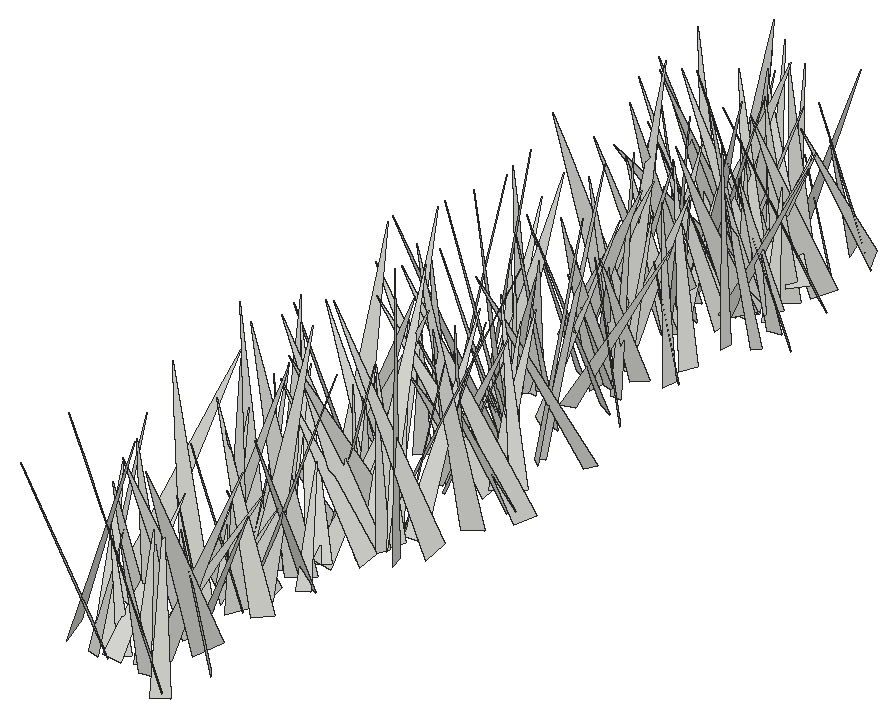
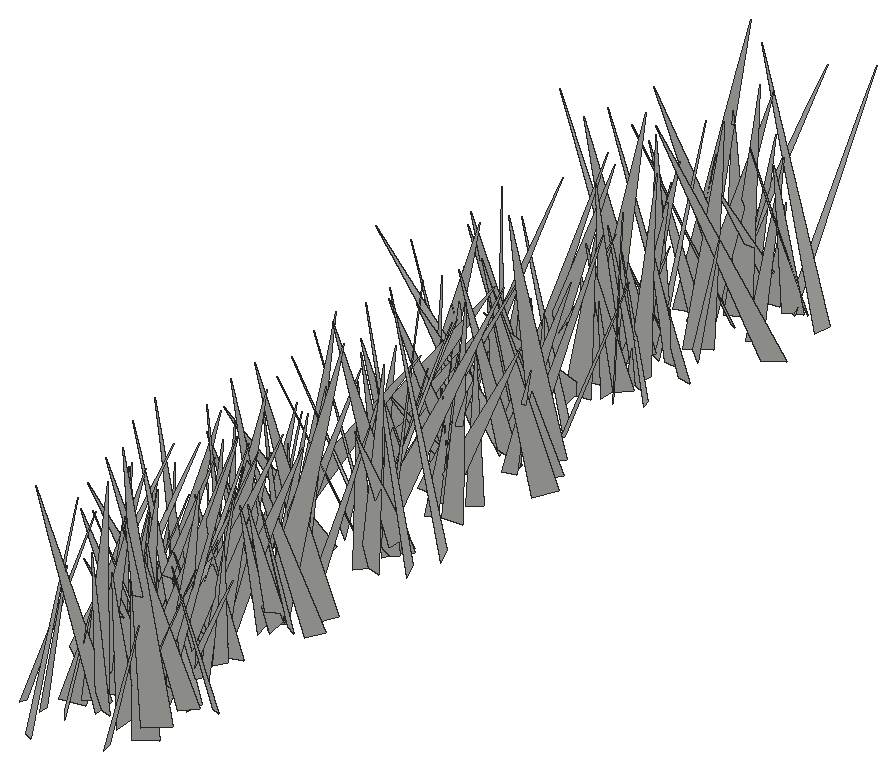
# SketchUp Ruby script. Lengths in inches.
U = 1.inch
M = Sketchup.active_model
def pt(a) = Geom::Point3d.new(a.map { |v| v * U })
def face(e, loops, mat)
  f = e.add_face(loops[0].map { |a| pt(a) })
  loops[1..].each { |l| e.add_face(l.map { |a| pt(a) }).erase! }
  f.material = f.back_material = mat if mat
  f
end
# faces: each face lists its corners as indices into pts; further lists are holes
def faces(e, pts, list, mat = nil) = list.each { |f| face(e, (f[0].is_a?(Array) ? f : [f]).map { |l| l.map { |i| pts[i] } }, mat) }
# xy, xz, yz: faces in a plane at the given z, y or x. An outline is a flat list of corners, or four numbers for a rectangle; further outlines are holes
def ring(l) = l.size == 4 ? [[l[0], l[1]], [l[2], l[1]], [l[2], l[3]], [l[0], l[3]]] : l.each_slice(2).to_a
def flat(e, list, mat, &to3) = list.each { |f| face(e, (f[0].is_a?(Array) ? f : [f]).map { |l| ring(l).map { |u, v| to3.(u, v) } }, mat) }
def xy(e, z, list, mat = nil) = flat(e, list, mat) { |x, y| [x, y, z] }
def xz(e, y, list, mat = nil) = flat(e, list, mat) { |x, z| [x, y, z] }
def yz(e, x, list, mat = nil) = flat(e, list, mat) { |y, z| [x, y, z] }
def lines(e, pts, list) = list.each { |a, b| e.add_line(pt(pts[a]), pt(pts[b])) }
# prism: a flat outline (further loops are holes) pulled along v
def prism(e, loops, v, mat = nil)
  f = face(e, loops, mat); d = Geom::Vector3d.new(v.map { |x| x * U })
  f.pushpull(f.normal.samedirection?(d) ? d.length : -d.length)
end
def box(e, o, s, mat = nil) = prism(e, [[o, [o[0] + s[0], o[1], o[2]], [o[0] + s[0], o[1] + s[1], o[2]], [o[0], o[1] + s[1], o[2]]]], [0, 0, s[2]], mat)
def at(x, y, z, deg = 0) = Geom::Transformation.translation(pt([x, y, z])) * Geom::Transformation.rotation(ORIGIN, Z_AXIS, deg.degrees)
def axes(o, x, y, z) = Geom::Transformation.new([*x, 0, *y, 0, *z, 0, *pt(o).to_a, 1])
def part(name) = M.definitions.add(name)
# library, detail: a bought-in or finely detailed component or shape, given as its bounding box
def library(name, o, s) = part(name).tap { |d| box(d.entities, o, s) }
def detail(e, o, s) = box(e.add_group.entities, o, s)
def put(e, d, t, mat = nil) = e.add_instance(d, t).tap { |i| i.material = mat if mat }
def group(e, t, mat = nil) = e.add_group.tap { |g| g.transformation = t; g.material = mat if mat }.entities
root = M.entities
c1 = part("fur_instance\#9")
p = [[0.8125,0,1.79],[0.67,-0.02,1.48],[0,-0.11,0],[0,0.11,0]]
faces(c1.entities,p,[[0,1,2,3]])
put(root,c1,axes([148.79,14.21,-27.1],[-4.50054,-5.78959,0.45114],[-5.68851,4.51005,1.13049],[1.1678,-0.3432,7.24542]))
put(root,c1,axes([154.44,11.93,-27.1],[-3.13208,3.88614,1.48189],[4.03166,3.29255,-0.11327],[1.02167,-1.07935,4.98991]))
put(root,c1,axes([152.23,13.52,-27.1],[0.17037,-4.40384,1.04145],[-4.5148,-0.2364,-0.26107],[-0.30825,1.02847,4.3994]))
put(root,c1,axes([153.88,12.75,-27.1],[-6.31099,-5.2237,1.0112],[-5.28027,5.95593,-2.18722],[-0.65451,2.31907,7.89505]))
put(root,c1,axes([146.15,14.9,-27.1],[7.97506,1.59703,0.67128],[1.71117,-7.75527,-1.87893],[-0.27022,-1.97686,7.91339]))
put(root,c1,axes([153.12,17.74,-27.1],[6.488,-4.94571,0.82766],[-4.48999,-6.33233,-2.64212],[-2.23271,-1.63731,7.71838]))
put(root,c1,axes([150.02,14.4,-27.1],[-1.79664,3.17113,0.9039],[3.29721,1.71578,0.53432],[-0.03822,-1.04932,3.60534]))
put(root,c1,axes([151.32,14.3,-27.1],[-2.54986,2.80817,1.27437],[2.87177,2.76487,-0.34653],[1.12374,-0.69377,3.77724]))
put(root,c1,axes([154.86,15.79,-27.1],[-3.48684,-2.54111,1.02639],[-2.66037,3.53733,-0.28017],[0.65812,0.83597,4.30544]))
put(root,c1,axes([148.54,14.46,-27.1],[-2.22109,4.73282,1.14399],[4.81333,2.32397,-0.26934],[0.73496,-0.91711,5.22114]))
put(root,c1,axes([150.7,16.51,-27.1],[3.54462,-5.56954,2.15269],[-5.7416,-3.86654,-0.54956],[-1.63946,1.49942,6.57891]))
put(root,c1,axes([149.64,13.77,-27.1],[-1.38897,4.86037,0.26759],[4.61521,1.40338,-1.53442],[1.54748,0.17706,4.81643]))
put(root,c1,axes([151.85,15.16,-27.1],[6.12264,-2.56902,1.18593],[-2.80714,-5.86992,1.77677],[-0.35534,2.10644,6.39763]))
put(root,c1,axes([151.7,18.47,-27.1],[4.33462,-5.23656,1.50263],[-4.77333,-4.57611,-2.17783],[-2.62578,-0.3257,6.43953]))
put(root,c1,axes([148.57,13.49,-27.1],[3.46655,5.88623,0.70358],[5.62008,-3.5225,1.77941],[-1.8861,0.32244,6.59533]))
put(root,c1,axes([148.3,18.06,-27.1],[-4.48343,0.78051,2.64752],[1.64873,4.80743,1.37477],[2.21365,-1.99978,4.33824]))
put(root,c1,axes([150.24,17.51,-27.1],[4.10846,4.74791,0.21399],[4.46685,-3.7608,-2.31765],[1.62348,-1.66782,5.83529]))
put(root,c1,axes([151.82,18.53,-27.1],[5.27208,0.02621,0.0042],[0.02652,-5.23568,-0.61848],[-0.0011,-0.61849,5.23574]))
put(root,c1,axes([151.16,19.8,-27.1],[-2.98198,-2.20876,0.85448],[-2.34628,2.94214,-0.58291],[0.32208,0.98295,3.66484]))
put(root,c1,axes([151.24,22.88,-27.1],[-4.09949,-5.26965,1.04192],[-4.89422,4.20438,2.00758],[2.21389,-0.46331,6.36747]))
put(root,c1,axes([150.1,20.66,-27.1],[-5.03128,5.10175,2.45438],[5.52933,5.13327,0.66454],[1.21582,-2.23324,7.13442]))
put(root,c1,axes([146.08,19.17,-27.1],[0.28527,8.21503,1.11931],[7.94931,0.04717,-2.37217],[2.35543,-1.15413,7.87026]))
put(root,c1,axes([149.73,21.37,-27.1],[1.87721,3.55983,2.07479],[3.45548,-2.60202,1.33802],[-2.2443,-1.02868,3.79553]))
put(root,c1,axes([153.16,22.39,-27.1],[1.40362,-5.52471,3.15038],[-5.88186,-2.35471,-1.50878],[-2.41887,2.51999,5.49692]))
put(root,c1,axes([151.72,21.93,-27.1],[-6.82221,1.72842,2.33339],[1.55801,7.20655,-0.7829],[2.45045,0.23004,6.99407]))
put(root,c1,axes([150.13,22.43,-27.1],[2.36408,2.77163,0.06713],[2.67068,-2.25294,-1.03299],[0.74428,-0.71945,3.49339]))
put(root,c1,axes([150.95,24.84,-27.1],[-1.08369,-5.40972,1.03151],[-5.49173,1.14023,0.21038],[0.41232,0.96864,5.51318]))
put(root,c1,axes([152.11,24.91,-27.1],[-3.71284,-0.24914,0.82183],[0.046,3.58403,1.29433],[0.85753,-1.27095,3.48884]))
put(root,c1,axes([152.89,26.65,-27.1],[-1.67702,-6.45132,0.05531],[-6.32349,1.655,1.30744],[1.27907,-0.27646,6.53625]))
put(root,c1,axes([148.5,23.88,-27.1],[4.58596,6.39713,1.96066],[6.63658,-4.04695,-2.31874],[0.85046,-2.91504,7.52182]))
put(root,c1,axes([151.08,24.09,-27.1],[7.89024,2.57718,0.73013],[2.64489,-7.85516,-0.85554],[-0.42369,-1.04189,8.25626]))
put(root,c1,axes([150,22.96,-27.1],[0.07202,5.27236,0.64208],[5.29211,-0.12578,0.43929],[-0.45123,-0.63374,5.25452]))
put(root,c1,axes([151.84,23.54,-27.1],[6.54564,-3.57049,3.76512],[-4.66006,-6.71077,1.73761],[-2.28219,3.46223,7.25083]))
put(root,c1,axes([152.01,27.12,-27.1],[2.92408,-7.38877,2.72238],[-7.56214,-3.44459,-1.22649],[-2.19528,2.02396,7.85111]))
put(root,c1,axes([150.25,25.65,-27.1],[-7.50799,1.69583,1.59774],[1.55933,7.66276,-0.80567],[1.73121,0.45255,7.65484]))
put(root,c1,axes([153.1,25.97,-27.1],[-2.61192,2.51011,0.78878],[2.46687,2.72278,-0.49597],[0.91509,-0.17543,3.58843]))
put(root,c1,axes([148.5,27.18,-27.1],[3.90059,1.73334,0.99556],[1.91928,-3.85762,-0.80331],[-0.55855,-1.15086,4.19211]))
put(root,c1,axes([149.73,26.11,-27.1],[1.82838,5.64567,1.15342],[5.69001,-1.95997,0.57384],[-0.90985,-0.91206,5.90655]))
put(root,c1,axes([150.32,27.71,-27.1],[-4.40906,-3.22075,2.19411],[-3.50304,4.72714,-0.10035],[1.70765,1.38134,5.45921]))
put(root,c1,axes([150.4,26.9,-27.1],[-3.17134,4.85922,0.78552],[4.77597,3.26378,-0.90795],[1.19131,-0.14895,5.73106]))
put(root,c1,axes([150.79,27.14,-27.1],[-7.20595,2.28011,2.02761],[1.9171,7.42879,-1.54068],[2.37378,0.922,7.39939]))
put(root,c1,axes([153.77,30.75,-27.1],[-5.93019,0.58333,0.46706],[0.68124,5.75556,1.46115],[0.30714,-1.50292,5.77689]))
put(root,c1,axes([153.27,31.49,-27.1],[-6.87965,3.10007,2.46286],[3.78941,6.58637,2.29475],[1.14737,-3.16466,7.18848]))
put(root,c1,axes([151.9,28.78,-27.1],[-2.77056,6.19265,0.76015],[6.19361,2.62958,1.15202],[-0.75223,-1.15721,6.68563]))
put(root,c1,axes([152.33,34.43,-27.1],[-7.59167,-1.95799,2.55179],[-0.44126,7.11339,4.14535],[3.18601,-3.68034,6.65457]))
put(root,c1,axes([149.74,32.8,-27.1],[-4.13984,-2.04423,0.54277],[-1.65039,3.86825,1.98107],[1.32277,-1.57147,4.17043]))
put(root,c1,axes([150.23,31.9,-27.1],[5.73054,2.09287,1.0832],[2.24178,-5.71944,-0.8093],[-0.7265,-1.14039,6.04684]))
put(root,c1,axes([156,33.73,-27.1],[-8.03194,-0.35365,0.82088],[-0.22203,7.97883,1.26494],[0.86581,-1.23463,7.93959]))
put(root,c1,axes([153.75,32.03,-27.1],[-4.82421,0.67017,1.12309],[0.52178,4.9221,-0.69578],[1.19925,0.5543,4.82058]))
put(root,c1,axes([152.2,31.63,-27.1],[0.68638,4.30492,0.85677],[4.11958,-0.93113,1.37825],[-1.51508,-0.58153,4.13569]))
put(root,c1,axes([152.04,28.875,-27.1],[-5.06896,3.36354,0.19703],[2.56301,4.08037,-3.71862],[2.18706,3.01393,4.81452]))
put(root,c1,axes([155.05,31.53,-27.1],[-7.31055,-2.64435,2.80127],[-3.45475,7.15889,-2.25809],[1.70424,3.16886,7.43894]))
put(root,c1,axes([153.93,33,-27.1],[-4.87029,1.64927,0.93909],[1.65484,4.95663,-0.12272],[0.92923,-0.18296,5.1405]))
put(root,c1,axes([150.76,34.07,-27.1],[2.98723,-2.64764,1.00912],[-2.72025,-3.09017,-0.05514],[-0.79284,0.62671,3.99131]))
put(root,c1,axes([150.45,34.98,-27.1],[-3.80657,-5.75041,0.9295],[-5.82495,3.76407,-0.56819],[0.03325,1.08891,6.87272]))
put(root,c1,axes([152.98,31.97,-27.1],[-2.31741,7.72302,0.72504],[7.71845,2.37113,-0.58682],[0.77216,-0.52327,8.04183]))
put(root,c1,axes([151.19,35.68,-27.1],[-5.49496,2.98551,0.84144],[3.09795,5.36781,1.18541],[0.15494,-1.44541,6.14025]))
put(root,c1,axes([149.84,36.91,-27.1],[0.38747,-3.62863,0.53891],[-3.66751,-0.39531,-0.02484],[-0.08219,0.53319,3.64917]))
put(root,c1,axes([152.91,34.04,-27.1],[-5.36407,2.31527,0.60969],[2.0889,5.25672,-1.5839],[1.1699,1.22955,5.6236]))
put(root,c1,axes([153.18,34.7,-27.1],[3.77893,2.89431,1.05154],[2.64296,-3.90266,1.24382],[-1.58036,0.3941,4.59459]))
put(root,c1,axes([147.38,36.65,-27.1],[1.67696,-6.87357,2.26471],[-6.67493,-0.57073,3.21041],[2.79647,2.7596,6.30488]))
put(root,c1,axes([148.57,35.34,-27.1],[-4.94866,6.16749,2.69055],[6.18584,5.48419,-1.19385],[2.6481,-1.28527,7.81677]))
put(root,c1,axes([156.03,36.91,-27.1],[-0.49595,7.7495,2.67586],[7.77568,-0.40515,2.61451],[-2.59882,-2.6911,7.31198]))
put(root,c1,axes([154.18,34.14,-27.1],[-5.33853,3.8285,0.2094],[3.37353,4.86067,-2.86257],[1.82225,2.21756,5.91295]))
put(root,c1,axes([149.52,37.68,-27.1],[-2.08975,2.94897,0.92989],[3.09202,1.98432,0.65582],[-0.0238,-1.13764,3.55435]))
put(root,c1,axes([146.56,38.29,-27.1],[5.35038,-4.23141,0.69897],[-4.27634,-5.17862,1.38378],[0.32603,1.51562,6.67957]))
put(root,c1,axes([151.71,35.46,-27.1],[7.40987,3.38689,0.1989],[3.26816,-7.25381,1.76579],[-0.91088,1.52574,7.95356]))
put(root,c1,axes([151.6,38.6,-27.1],[5.88028,2.97965,0.94292],[3.11911,-5.72141,-1.37172],[-0.19635,-1.65292,6.44782]))
put(root,c1,axes([153.2,39.57,-27.1],[-2.5079,-4.6968,1.95628],[-4.90602,2.8103,0.45782],[1.34828,1.48955,5.3047]))
put(root,c1,axes([151.51,40.9,-27.1],[5.83634,-0.86723,1.56304],[-0.35494,-5.79341,-1.88904],[-1.75191,-1.71533,5.58985]))
put(root,c1,axes([154.13,40.99,-27.1],[-6.77007,0.71674,0.61078],[0.8862,6.3486,2.37288],[0.31848,-2.42944,6.38099]))
put(root,c1,axes([156.48,39.6875,-27.1],[-2.71557,-5.16024,0.69315],[-4.67023,2.06855,-2.89705],[-2.30163,1.89099,5.06058]))
put(root,c1,axes([150.57,36.36,-27.1],[0.71123,8.26754,0.30404],[8.18462,-0.74766,1.1847],[-1.20692,-0.19821,8.21307]))
put(root,c1,axes([157.59,39.53,-27.1],[-2.51256,7.06983,2.10699],[6.38069,0.96553,4.36915],[-3.70253,-3.13371,6.09968]))
put(root,c1,axes([151.29,39.43,-27.1],[5.01849,-2.22986,0.6447],[-2.32023,-4.77497,1.54574],[0.06662,1.67347,5.26955]))
put(root,c1,axes([151.8,42.02,-27.1],[1.73038,-3.85975,0.19684],[-3.59553,-1.68683,-1.46882],[-1.41726,-0.43309,3.96667]))
put(root,c1,axes([148.7,41.67,-27.1],[2.93376,-3.22318,1.07266],[-3.3076,-3.03341,-0.06853],[-0.77414,0.74566,4.35788]))
put(root,c1,axes([152.27,39.12,-27.1],[3.66299,2.22216,0.32756],[1.7102,-3.16536,2.34915],[-1.4562,1.87225,3.58288]))
put(root,c1,axes([150.45,42.58,-27.1],[-4.33976,4.07233,1.17149],[4.17045,3.80756,2.21352],[-0.75076,-2.38923,5.52429]))
put(root,c1,axes([149.81,44.04,-27.1],[4.21418,-1.38432,0.79636],[-0.98829,-4.02576,-1.76817],[-1.25452,-1.47878,4.06808]))
put(root,c1,axes([150.1,42.12,-27.1],[-2.43911,-2.15453,1.73505],[-2.51562,2.68975,-0.19638],[1.15067,1.31336,3.24849]))
put(root,c1,axes([151.35,41,-27.1],[-1.53438,4.71255,0.03454],[4.47921,1.44703,1.55125],[-1.46492,-0.51147,4.70702]))
put(root,c1,axes([148.62,43.75,-27.1],[0.4786,-6.17329,1.68247],[-6.39725,-0.42884,0.2463],[0.12453,1.69584,6.18692]))
put(root,c1,axes([152.39,44.09,-27.1],[-3.30387,-7.05223,0.96215],[-6.92829,2.9435,-2.21582],[-1.63048,1.78244,7.4659]))
put(root,c1,axes([155.22,41.9,-27.1],[-1.00856,5.27208,0.80529],[5.17147,0.76643,1.45913],[-1.30357,-1.0384,5.16556]))
put(root,c1,axes([154.33,41.08,-27.1],[-4.2837,1.86088,0.37109],[1.60299,4.03921,-1.75094],[1.01537,1.47394,4.32979]))
put(root,c1,axes([152.76,44.19,-27.1],[-3.61548,-1.81279,0.7212],[-1.71327,3.67656,0.65243],[0.9333,-0.2734,3.99152]))
put(root,c1,axes([153.51,42.05,-27.1],[-2.74828,4.07366,1.32335],[3.94461,3.01992,-1.10419],[1.66916,-0.42944,4.78838]))
put(root,c1,axes([153.38,43.69,-27.1],[-5.70122,-3.26457,0.62497],[-3.32356,5.6155,-0.98593],[0.04408,1.16649,6.49533]))
put(root,c1,axes([152.47,44.92,-27.1],[-6.0406,-4.0795,1.11122],[-4.22494,5.74856,-1.86274],[-0.16426,2.16279,7.04708]))
put(root,c1,axes([156.71,46.26,-27.1],[-1.84266,-5.86998,0.99209],[-5.21002,1.08759,-3.24178],[-2.88039,1.78795,5.22904]))
put(root,c1,axes([152.79,44.46,-27.1],[-4.924,0.48292,1.1816],[0.20052,4.94285,-1.18453],[1.26062,1.10005,4.80373]))
put(root,c1,axes([150.9,46.14,-27.1],[-6.29622,-3.82649,2.40942],[-4.00808,6.63484,0.06324],[2.09347,1.19444,7.36752]))
put(root,c1,axes([146.57,47.02,-27.1],[7.04246,3.4796,1.7186],[3.70112,-7.09298,-0.80545],[-1.16744,-1.49647,7.81378]))
put(root,c1,axes([154.09,44.84,-27.1],[4.5947,4.98178,1.41698],[4.55399,-4.78808,2.06705],[-2.46722,0.43974,6.4542]))
put(root,c1,axes([148.83,48.7,-27.1],[5.31861,-1.95589,0.12332],[-1.94358,-5.30997,-0.39374],[-0.25139,-0.32717,5.65315]))
put(root,c1,axes([152.53,48.37,-27.1],[-3.42492,-4.02626,1.68032],[-4.34426,2.9504,-1.78518],[-0.40205,2.41841,4.97534]))
put(root,c1,axes([148.8,48.79,-27.1],[-2.37433,3.47563,1.70417],[3.72029,2.6012,-0.12184],[1.06942,-1.33243,4.20745]))
put(root,c1,axes([148.57,48.26,-27.1],[-1.59502,6.99566,2.35908],[7.02793,2.17795,-1.70682],[2.26111,-1.83463,6.96922]))
put(root,c1,axes([146.97,49.47,-27.1],[7.03431,3.48518,2.0857],[3.73576,-7.18871,-0.58711],[-1.59396,-1.46769,7.82836]))
put(root,c1,axes([154.09,45.27,-27.1],[4.35175,7.0169,0.44581],[6.16578,-4.0605,3.72408],[-3.37917,1.6275,7.36925]))
put(root,c1,axes([149.11,50.8125,-27.1],[4.27597,-2.96302,0.67606],[-2.94629,-4.32773,-0.33261],[-0.74558,0.10858,5.19161]))
put(root,c1,axes([153.36,51.72,-27.1],[-2.96525,-5.05492,0.58848],[-5.08807,2.93137,-0.45808],[-0.10025,0.73898,5.84252]))
put(root,c1,axes([151.42,48.41,-27.1],[3.77289,4.9439,0.17652],[4.9129,-3.7705,0.5956],[-0.58026,0.22179,6.19049]))
put(root,c1,axes([148.54,48.08,-27.1],[-4.13598,4.27474,0.09369],[4.07434,3.97972,-1.71759],[1.29691,1.13001,5.6947]))
put(root,c1,axes([148.81,50.61,-27.1],[-1.16984,-6.03511,2.92768],[-6.70455,0.96018,-0.69968],[-0.2073,3.00298,6.1075]))
put(root,c1,axes([151.54,53.79,-27.1],[6.17469,-3.94346,0.96595],[-3.5616,-6.10514,-2.15707],[-1.94909,-1.33681,7.00177]))
put(root,c1,axes([154.96,50.93,-27.1],[-3.71707,-2.68533,1.32909],[-2.9797,3.53518,-1.19076],[0.31439,1.75658,4.42828]))
put(root,c1,axes([151.91,53.7,-27.1],[-0.76321,-4.71965,0.1503],[-4.6984,0.77422,0.45372],[0.47201,0.07524,4.75939]))
put(root,c1,axes([151.09,54.35,-27.1],[-0.50575,-5.47671,0.42869],[-5.44927,0.55465,0.65709],[0.69543,0.36321,5.46062]))
put(root,c1,axes([151.54,50.71,-27.1],[5.52796,-0.81869,0.7417],[-1.07099,-4.89962,2.57397],[-0.27083,2.66498,4.96017]))
put(root,c1,axes([149.9,53.875,-27.1],[-2.91722,-4.26379,0.81225],[-4.33997,2.88016,-0.46811],[0.06569,0.93518,5.14499]))
put(root,c1,axes([152.88,55.31,-27.1],[2.25117,-4.50739,0.41367],[-4.42833,-2.28883,-0.84056],[-0.93676,-0.01195,4.96767]))
put(root,c1,axes([149.66,56.09,-27.1],[4.03439,-1.67825,0.01541],[-1.64329,-3.95818,-0.85174],[-0.3411,-0.78061,4.28572]))
put(root,c1,axes([152.96,53.1,-27.1],[2.80201,6.02167,1.40008],[5.6342,-3.12002,2.14317],[-2.54489,-0.27744,6.28638]))
put(root,c1,axes([147.13,56.52,-27.1],[3.33833,-6.51025,0.54896],[-6.14625,-2.92038,2.74304],[2.21549,1.70799,6.78259]))
put(root,c1,axes([151.29,55.73,-27.1],[-5.71627,0.02456,1.51927],[0.09668,5.9079,0.26822],[1.51639,-0.28405,5.71003]))
put(root,c1,axes([149.28,58.49,-27.1],[5.28612,-6.00356,2.19792],[-5.60526,-5.72373,-2.15328],[-3.07484,0.113,7.70384]))
put(root,c1,axes([154.4375,56.58,-27.1],[-2.57629,-2.49445,0.93197],[-2.62206,2.60252,-0.28257],[0.46438,0.85602,3.57488]))
put(root,c1,axes([154.34,55.99,-27.1],[-5.10853,0.04095,1.59169],[-0.11644,5.32521,-0.51071],[1.58796,0.52222,5.08311]))
put(root,c1,axes([151.6,55.68,-27.1],[1.45734,4.18221,0.34787],[4.02467,-1.49715,1.13854],[-1.18907,0.05834,4.28]))
put(root,c1,axes([146.54,58.17,-27.1],[2.73482,-5.11249,1.4467],[-5.08402,-2.04521,2.38319],[1.54377,2.32148,5.28557]))
put(root,c1,axes([149.5625,58.36,-27.1],[-0.77235,4.89048,2.70767],[4.92537,1.88806,-2.00519],[2.64368,-2.08884,4.52687]))
put(root,c1,axes([154.05,58.01,-27.1],[-5.59826,1.4556,0.99849],[1.35798,5.67289,-0.65612],[1.12768,0.39476,5.74707]))
put(root,c1,axes([147.93,58.52,-27.1],[1.92341,3.31368,0.82854],[3.39872,-1.95136,-0.08567],[-0.34002,-0.7604,3.83049]))
put(root,c1,axes([150.875,60.37,-27.1],[-1.01411,-6.0227,1.51425],[-5.97973,0.53295,-1.88497],[-1.67593,1.7428,5.80932]))
put(root,c1,axes([149.61,57.83,-27.1],[1.82525,7.99707,1.79582],[8.16577,-1.93273,0.30716],[-0.70587,-1.67961,8.19697]))
put(root,c1,axes([150.9375,60.5625,-27.1],[4.1746,-2.61988,2.8232],[-2.37692,-5.02847,-1.15163],[-3.03059,0.33503,4.79215]))
put(root,c1,axes([148.71,58.82,-27.1],[5.15508,0.33774,1.32609],[0.02228,-5.18864,1.23487],[-1.36825,1.188,5.01637]))
put(root,c1,axes([149,58.4,-27.1],[-5.03448,1.97141,0.87824],[1.57247,4.87743,-1.93439],[1.47821,1.52579,5.04882]))
put(root,c1,axes([150.87,60.31,-27.1],[5.91365,2.78735,2.33328],[2.94924,-6.28377,0.03183],[-2.12497,-0.96423,6.53755]))
put(root,c1,axes([149.22,59.25,-27.1],[-5.01986,0.40192,1.5189],[-0.17545,4.90978,-1.87904],[1.56135,1.84392,4.67223]))
put(root,c1,axes([149.47,63.62,-27.1],[2.6009,-7.25193,0.96085],[-7.2129,-2.71231,-0.94648],[-1.21974,0.57558,7.64587]))
put(root,c1,axes([149.94,62.52,-27.1],[4.17117,1.8451,1.43695],[2.27213,-3.89306,-1.59669],[-0.55375,-2.07548,4.27243]))
put(root,c1,axes([152.65,64.55,-27.1],[3.73251,-5.71066,0.85994],[-5.41751,-3.81707,-1.83396],[-2.00044,-0.31799,6.57114]))
put(root,c1,axes([154.13,61.12,-27.1],[-5.50715,-0.70612,1.61288],[-1.08889,5.52799,-1.29784],[1.38358,1.53996,5.39842]))
put(root,c1,axes([152.49,62.82,-27.1],[-7.29173,-1.24054,0.1592],[-1.24954,7.26646,-0.60898],[0.05425,0.6271,7.37139]))
put(root,c1,axes([149.73,68.3125,-28.22],[5.96387,-5.74764,0.45925],[-4.68382,-5.21453,-4.43673],[-3.36276,-2.93042,6.99418]))
put(root,c1,axes([148.23,62.89,-27.1],[0.29151,4.89673,1.62599],[5.06271,0.04273,-1.03633],[0.99541,-1.65136,4.79468]))
put(root,c1,axes([153.89,63.66,-27.1],[-3.07283,-1.79032,0.75021],[-1.87261,3.10397,-0.26279],[0.51124,0.60869,3.54662]))
put(root,c1,axes([150.5,66.25,-28.22],[-4.50054,-5.78959,0.45114],[-5.68851,4.51005,1.13049],[1.1678,-0.3432,7.24542]))
put(root,c1,axes([155.55,62,-27.1],[-6.80362,-1.51626,0.05987],[-1.39466,6.13985,-2.9915],[-0.59797,2.93174,6.29597]))
put(root,c1,axes([149.56,64.02,-28.22],[-3.61019,-4.99925,2.09321],[-5.40705,3.49453,-0.97958],[0.37125,2.28107,6.08822]))
put(root,c1,axes([148.56,63.84,-27.1],[-3.29969,1.99263,1.18367],[2.06312,3.46364,-0.07948],[1.05601,-0.54058,3.85386]))
put(root,c1,axes([152.93,65.66,-27.1],[-3.89152,-1.38284,0.09587],[-1.31779,3.77936,1.02238],[0.42995,-0.93252,4.00136]))
put(root,c1,axes([153.84,65.64,-27.1],[3.33283,-3.55166,1.19436],[-3.37517,-3.53973,-1.10774],[-1.62758,0.06765,4.74288]))
put(root,c1,axes([152.64,65.57,-27.1],[-3.58815,0.95471,1.93369],[1.59157,3.70529,1.12394],[1.45517,-1.69849,3.5388]))
put(root,c1,axes([148.56,66.01,-27.1],[7.85727,-0.11013,0.63762],[0.0287,-7.70188,-1.68396],[-0.64642,-1.6806,7.67549]))
put(root,c1,axes([149.99,62.93,-27.1],[0.7,4.04155,0.09862],[4.02713,-0.70587,0.34334],[-0.35517,-0.03822,4.08733]))
put(root,c1,axes([152.1,63.36,-27.1],[5.39304,-0.33096,0.39775],[-0.43435,-5.15892,1.59671],[-0.28121,1.6213,5.16187]))
put(root,c1,axes([153.9375,65.5625,-28.22],[0.17037,-4.40384,1.04145],[-4.5148,-0.2364,-0.26107],[-0.30825,1.02847,4.3994]))
put(root,c1,axes([155.59,64.8,-28.22],[-6.31099,-5.2237,1.0112],[-5.28027,5.95593,-2.18722],[-0.65451,2.31907,7.89505]))
put(root,c1,axes([152.02,65.38,-27.1],[3.93082,-2.70083,1.38603],[-2.7651,-4.12134,-0.18897],[-1.2529,0.6221,4.76552]))
put(root,c1,axes([149.59,66.04,-28.22],[-2.11494,-3.26023,0.3236],[-3.25153,2.04149,-0.68318],[-0.40176,0.64034,3.82562]))
put(root,c1,axes([149.86,67.28,-27.1],[-1.24664,-7.42641,1.30497],[-7.49381,1.07378,-1.04811],[-0.83512,1.45053,7.45702]))
put(root,c1,axes([152.46,66.47,-27.1],[-7.15146,0.58689,0.88826],[0.71619,7.11549,1.06478],[0.78773,-1.14116,7.09606]))
put(root,c1,axes([147.86,66.95,-28.22],[7.97506,1.59703,0.67128],[1.71117,-7.75527,-1.87893],[-0.27022,-1.97686,7.91339]))
put(root,c1,axes([155.46,67.88,-27.1],[-4.1792,-5.61615,0.15739],[-5.61189,4.16336,-0.45249],[-0.26934,0.3962,6.98585]))
put(root,c1,axes([150.02,68.97,-28.22],[0.33917,-8.30019,0.61155],[-8.21231,-0.43312,-1.32383],[-1.35096,0.54903,8.20095]))
put(root,c1,axes([151.73,66.4375,-28.22],[-1.79664,3.17113,0.9039],[3.29721,1.71578,0.53432],[-0.03822,-1.04932,3.60534]))
put(root,c1,axes([150.67,64.89,-27.1],[-7.44461,1.33123,0.56849],[1.18187,7.30967,-1.63995],[0.83578,1.52121,7.38274]))
put(root,c1,axes([146.73,66.49,-28.22],[2.48119,3.58815,0.88423],[3.68479,-2.32113,-0.92071],[0.2811,-1.24521,4.2642]))
put(root,c1,axes([153.03,66.35,-28.22],[-2.54986,2.80817,1.27437],[2.87177,2.76487,-0.34653],[1.12374,-0.69377,3.77724]))
put(root,c1,axes([150.25,66.5,-28.22],[-2.22109,4.73282,1.14399],[4.81333,2.32397,-0.26934],[0.73496,-0.91711,5.22114]))
put(root,c1,axes([152.41,68.55,-28.22],[3.54462,-5.56954,2.15269],[-5.7416,-3.86654,-0.54956],[-1.63946,1.49942,6.57891]))
put(root,c1,axes([151.35,65.81,-28.22],[-1.38897,4.86037,0.26759],[4.61521,1.40338,-1.53442],[1.54748,0.17706,4.81643]))
put(root,c1,axes([151.04,67.7,-27.1],[3.04965,-4.5466,3.26672],[-5.09549,-3.79519,-0.52522],[-2.31926,2.35973,5.44941]))
put(root,c1,axes([150.29,67.96,-27.1],[4.26333,-3.02404,0.31767],[-2.97687,-4.03955,1.49732],[0.61963,1.39963,5.00788]))
put(root,c1,axes([153.41,70.51,-28.22],[4.33462,-5.23656,1.50263],[-4.77333,-4.57611,-2.17783],[-2.62578,-0.3257,6.43953]))
put(root,c1,axes([150.28,65.54,-28.22],[3.46655,5.88623,0.70358],[5.62008,-3.5225,1.77941],[-1.8861,0.32244,6.59533]))
put(root,c1,axes([149.7,69.48,-27.1],[-4.06839,-1.50308,0.30492],[-1.46625,4.06536,0.47647],[0.44983,-0.34301,4.31092]))
put(root,c1,axes([149.56,67.47,-27.1],[4.3993,3.63087,0.47155],[3.65139,-4.40515,-0.14642],[-0.27004,-0.41338,5.70225]))
put(root,c1,axes([150.01,70.1,-28.22],[-4.48343,0.78051,2.64752],[1.64873,4.80743,1.37477],[2.21365,-1.99978,4.33824]))
put(root,c1,axes([146.75,68.8,-27.1],[1.17731,-6.81979,2.88625],[-6.91612,0.0321,2.89694],[2.64712,3.11697,6.28517]))
put(root,c1,axes([153.04,68.69,-27.1],[-3.19469,4.99874,1.10839],[5.10889,3.02549,1.08057],[-0.33936,-1.5103,5.83317]))
put(root,c1,axes([147.7,71.31,-28.22],[2.29516,-7.21123,1.1617],[-7.23425,-2.07612,1.40519],[1.00849,1.5189,7.43607]))
put(root,c1,axes([151.33,71.16,-27.1],[-3.30956,4.62511,3.28339],[5.43338,3.67626,0.29816],[1.62808,-2.86687,5.67942]))
put(root,c1,axes([148.1,69.6875,-28.22],[-1.99924,6.11191,2.2816],[6.3463,2.375,-0.80119],[1.51181,-1.88733,6.38047]))
put(root,c1,axes([146.87,71.42,-27.1],[-1.94061,6.26278,4.61542],[7.19839,3.24975,-1.38302],[2.95087,-3.80883,6.40903]))
put(root,c1,axes([154.31,73.625,-27.1],[-5.03232,-2.4099,0.87584],[-1.92345,4.82363,2.22078],[1.6956,-1.68045,5.11859]))
put(root,c1,axes([152.875,71.84,-28.22],[-2.98198,-2.20876,0.85448],[-2.34628,2.94214,-0.58291],[0.32208,0.98295,3.66484]))
put(root,c1,axes([150.43,71.51,-27.1],[6.68807,0.43229,0.66728],[0.41432,-6.71942,0.20043],[-0.67859,0.15798,6.69903]))
put(root,c1,axes([152.95,74.92,-28.22],[-4.09949,-5.26965,1.04192],[-4.89422,4.20438,2.00758],[2.21389,-0.46331,6.36747]))
put(root,c1,axes([149.6875,70.46,-28.22],[-6.09704,1.94582,1.05535],[1.61207,6.02238,-1.79053],[1.51697,1.42075,6.14444]))
put(root,c1,axes([150.3,71.81,-27.1],[0.9151,5.15761,1.58711],[5.35443,-1.06795,0.38322],[-0.67079,-1.48856,5.22413]))
put(root,c1,axes([152.88,73.68,-27.1],[3.69815,0.46024,1.83595],[1.02421,-3.87534,-1.09159],[-1.5917,-1.42435,3.56322]))
put(root,c1,axes([148.85,73.26,-28.22],[-3.57828,-1.18752,0.86435],[-1.11493,3.67791,0.43741],[0.95617,-0.15551,3.74473]))
